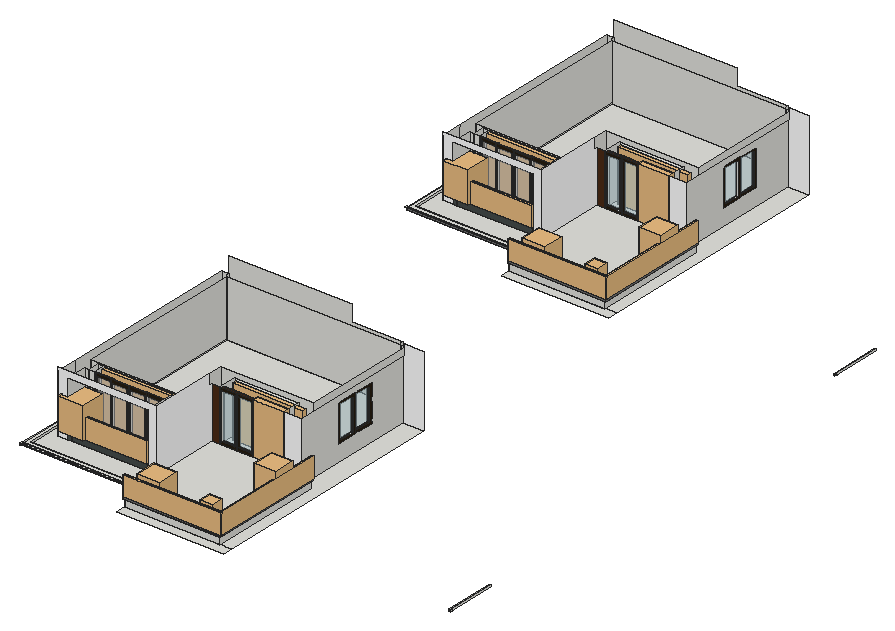
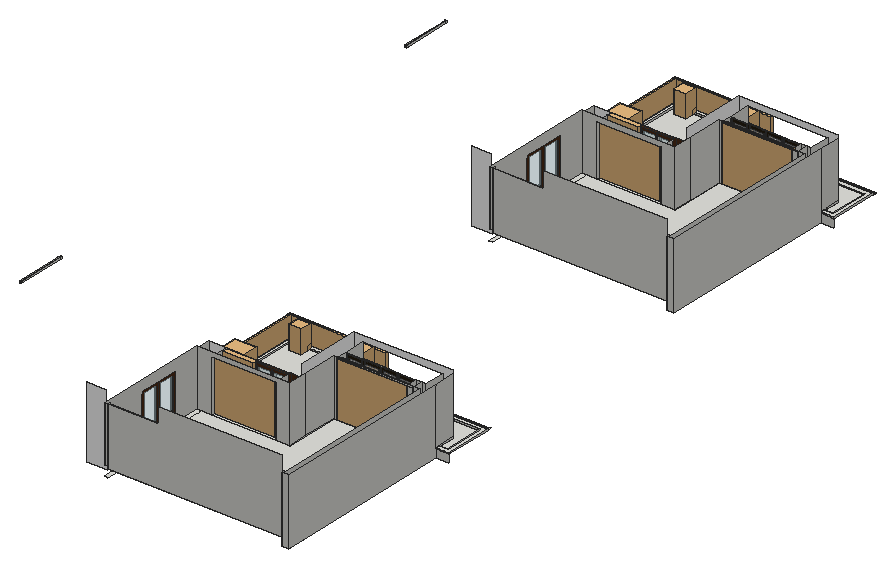
# SketchUp Ruby script. Lengths in inches.
U = 1.inch
M = Sketchup.active_model
def pt(a) = Geom::Point3d.new(a.map { |v| v * U })
def face(e, loops, mat)
  f = e.add_face(loops[0].map { |a| pt(a) })
  loops[1..].each { |l| e.add_face(l.map { |a| pt(a) }).erase! }
  f.material = f.back_material = mat if mat
  f
end
# faces: each face lists its corners as indices into pts; further lists are holes
def faces(e, pts, list, mat = nil) = list.each { |f| face(e, (f[0].is_a?(Array) ? f : [f]).map { |l| l.map { |i| pts[i] } }, mat) }
# xy, xz, yz: faces in a plane at the given z, y or x. An outline is a flat list of corners, or four numbers for a rectangle; further outlines are holes
def ring(l) = l.size == 4 ? [[l[0], l[1]], [l[2], l[1]], [l[2], l[3]], [l[0], l[3]]] : l.each_slice(2).to_a
def flat(e, list, mat, &to3) = list.each { |f| face(e, (f[0].is_a?(Array) ? f : [f]).map { |l| ring(l).map { |u, v| to3.(u, v) } }, mat) }
def xy(e, z, list, mat = nil) = flat(e, list, mat) { |x, y| [x, y, z] }
def xz(e, y, list, mat = nil) = flat(e, list, mat) { |x, z| [x, y, z] }
def yz(e, x, list, mat = nil) = flat(e, list, mat) { |y, z| [x, y, z] }
def lines(e, pts, list) = list.each { |a, b| e.add_line(pt(pts[a]), pt(pts[b])) }
# prism: a flat outline (further loops are holes) pulled along v
def prism(e, loops, v, mat = nil)
  f = face(e, loops, mat); d = Geom::Vector3d.new(v.map { |x| x * U })
  f.pushpull(f.normal.samedirection?(d) ? d.length : -d.length)
end
def box(e, o, s, mat = nil) = prism(e, [[o, [o[0] + s[0], o[1], o[2]], [o[0] + s[0], o[1] + s[1], o[2]], [o[0], o[1] + s[1], o[2]]]], [0, 0, s[2]], mat)
def at(x, y, z, deg = 0) = Geom::Transformation.translation(pt([x, y, z])) * Geom::Transformation.rotation(ORIGIN, Z_AXIS, deg.degrees)
def axes(o, x, y, z) = Geom::Transformation.new([*x, 0, *y, 0, *z, 0, *pt(o).to_a, 1])
def part(name) = M.definitions.add(name)
# library, detail: a bought-in or finely detailed component or shape, given as its bounding box
def library(name, o, s) = part(name).tap { |d| box(d.entities, o, s) }
def detail(e, o, s) = box(e.add_group.entities, o, s)
def put(e, d, t, mat = nil) = e.add_instance(d, t).tap { |i| i.material = mat if mat }
def group(e, t, mat = nil) = e.add_group.tap { |g| g.transformation = t; g.material = mat if mat }.entities
root = M.entities
M.materials.add("[Color M00]").color = [255, 255, 255]
M.materials.add("[Color M05]").color = [114, 114, 114]
M.materials.add("[Slate]").color = [70, 76, 75]
M.materials.add("[Translucent Glass Gray]2").color = [201, 201, 201]
M.materials["[Translucent Glass Gray]2"].alpha = 0.5
M.materials.add("[Translucent Glass Safety]").color = [204, 235, 244]
M.materials["[Translucent Glass Safety]"].alpha = 0.5
M.materials.add("[Wood Veneer 01]").color = [76, 44, 23]
M.materials.add("oak swatch").color = [40, 31, 19]
c1 = library("plant (1)",[-35.72,-28.42,0],[66.31,67.39,84.38])
c2 = library("Glass Railing",[0,0,0],[139.5,4.76,42])
c3 = part("Group\#6")
box(c3.entities,[0,0,0],[1.77,4.72,80.31],"oak swatch")
c4 = part("Exterior Sliding Doors")
xy(c4.entities,0,[[1.77,33.07,3.54,70.87],[1.77,70.87,3.54,108.66]])
xy(c4.entities,0,[[0,0,1.77,33.07],[0,108.66,1.77,141.73]],"oak swatch")
xy(c4.entities,4.72,[[0,4.72,1.77,33.07],[1.77,37.8,3.54,66.14],[1.77,75.88,3.54,103.9375],[0,108.66,1.77,137.01]],"oak swatch")
xy(c4.entities,75.59,[[1.77,37.8,3.54,66.14],[1.77,75.88,3.54,103.9375]])
xy(c4.entities,75.59,[[0,4.72,1.77,33.07],[0,108.66,1.77,137.01]],"oak swatch")
xy(c4.entities,80.31,[[0,0,1.77,33.07],[1.77,33.07,3.54,70.87],[1.77,70.87,3.54,108.66],[0,108.66,1.77,141.73]],"oak swatch")
xz(c4.entities,0,[[0,0,1.77,80.31]],"oak swatch")
xz(c4.entities,4.72,[[0,4.72,1.77,75.59]],"oak swatch")
xz(c4.entities,33.07,[[0,0,1.77,4.72],[1.77,0,3.54,80.31],[0,75.59,1.77,80.31]],"oak swatch")
xz(c4.entities,37.8,[[1.77,4.72,3.54,75.59]])
xz(c4.entities,66.14,[[1.77,4.72,3.54,75.59]],"oak swatch")
xz(c4.entities,70.87,[[1.77,0,3.54,80.31]])
xz(c4.entities,75.88,[[1.77,4.72,3.54,75.59]])
xz(c4.entities,103.9375,[[1.77,4.72,3.54,75.59]],"oak swatch")
xz(c4.entities,108.66,[[1.77,4.72,3.54,75.59]])
xz(c4.entities,108.66,[[0,0,3.54,4.72],[0,75.59,3.54,80.31]],"oak swatch")
xz(c4.entities,137.01,[[0,4.72,1.77,75.59]],"oak swatch")
xz(c4.entities,141.73,[[0,0,1.77,80.31]],"oak swatch")
yz(c4.entities,0,[[0,0,33.07,0,33.07,4.72,4.72,4.72,4.72,75.59,33.07,75.59,33.07,80.31,0,80.31],[108.66,0,141.73,0,141.73,80.31,108.66,80.31,108.66,75.59,137.01,75.59,137.01,4.72,108.66,4.72]],"oak swatch")
yz(c4.entities,1.77,[[4.72,4.72,33.07,75.59],[37.8,4.72,66.14,75.59],[75.88,4.72,103.9375,75.59],[108.66,4.72,137.01,75.59]],"[Translucent Glass Gray]2")
yz(c4.entities,1.77,[[0,0,33.07,0,33.07,4.72,4.72,4.72,4.72,75.59,33.07,75.59,33.07,80.31,0,80.31],[[33.07,0,70.87,80.31],[37.8,4.72,66.14,75.59]],[[70.87,0,141.73,80.31],[108.66,4.72,137.01,75.59],[75.88,4.72,103.9375,75.59]]],"oak swatch")
yz(c4.entities,3.54,[[[33.07,0,70.87,80.31],[37.8,4.72,66.14,75.59]],[[70.87,0,108.66,80.31],[75.88,4.72,103.9375,75.59]]],"oak swatch")
put(c4.entities,c3,at(0,33.07,0))
put(c4.entities,c3,at(0,103.9375,0))
c5 = library("Curtains",[0,0,0],[121.73,8.19,117.22])
c6 = library("Plant",[0,0,0],[12.59,12.59,14.16])
c7 = part("Group\#4")
g1 = group(c7.entities,at(0,0,0))
xy(g1,0,[[0,0,6,48]],"[Wood Veneer 01]")
xy(g1,4,[[0,4,1.8125,44],[1.8125,4,6,44]])
xy(g1,80,[[0,4,1.8125,44],[1.8125,4,6,44]])
xy(g1,84,[[0,0,6,48]],"[Wood Veneer 01]")
xz(g1,0,[[0,0,6,84]],"[Wood Veneer 01]")
xz(g1,4,[[0,4,1.8125,80],[1.8125,4,6,80]])
xz(g1,44,[[0,4,1.8125,80],[1.8125,4,6,80]])
xz(g1,48,[[0,0,6,84]],"[Wood Veneer 01]")
yz(g1,0,[[[0,0,48,84],[4,4,44,80]]],"[Wood Veneer 01]")
yz(g1,1.8125,[[4,4,44,80]],"[Translucent Glass Safety]")
yz(g1,6,[[[0,0,48,84],[4,4,44,80]]],"oak swatch")
g2 = group(c7.entities,at(0,48,0),"oak swatch")
xy(g2,0,[[0,0,6,48]],"[Wood Veneer 01]")
xy(g2,4,[[0,4,1.8125,44],[1.8125,4,6,44]])
xy(g2,80,[[0,4,1.8125,44],[1.8125,4,6,44]])
xy(g2,84,[[0,0,6,48]],"[Wood Veneer 01]")
xz(g2,0,[[0,0,6,84]],"[Wood Veneer 01]")
xz(g2,4,[[0,4,1.8125,80],[1.8125,4,6,80]])
xz(g2,44,[[0,4,1.8125,80],[1.8125,4,6,80]])
xz(g2,48,[[0,0,6,84]],"[Wood Veneer 01]")
yz(g2,0,[[[0,0,48,84],[4,4,44,80]]],"[Wood Veneer 01]")
yz(g2,1.8125,[[4,4,44,80]],"[Translucent Glass Safety]")
yz(g2,6,[[[0,0,48,84],[4,4,44,80]]],"oak swatch")
c8 = library("Flora+17",[-57.52,158.6,-38.64],[66.99,62.88,77.28])
c9 = library("modern+door",[0,0,0],[59.06,11.8125,86.61])
c10 = library("plant1",[-367.84,-375.82,-125.45],[750.59,696.16,1346.74])
c11 = part("skp4FF")
put(c11.entities,c10,at(0,0,0))
xy(root,121.3125,[[1384.3,481.81,1607.7,502.24],[1384.3,502.24,1583.39,538.49],[1583.39,502.24,1607.7,502.24,1607.7,1001.66,1563.95,1001.66,1563.95,738.06,1583.39,738.06],[1384.3,538.49,1583.39,638.99],[1172.33,638.99,1172.33,1021.31,1187.0625,1021.31,1187.0625,662.52,1204.64,662.52,1204.64,638.99],
  [1384.3,638.99,1583.39,738.06],[1204.64,648.22,1204.64,662.52,1364.27,662.52,1364.27,776.62,1373.95,776.62,1373.95,648.22],[1384.3,738.06,1563.95,749.87],[1548.25,813.85,1554.73,1021.31],[1384.3,1481.16,1607.7,1501.6],
  [1384.3,1501.6,1583.39,1537.85],[1583.39,1501.6,1607.7,1501.6,1607.7,2001.02,1563.95,2001.02,1563.95,1737.41,1583.39,1737.41],[1384.3,1537.85,1583.39,1638.35],[1172.33,1638.35,1172.33,2020.66,1187.0625,2020.66,1187.0625,1661.875,1204.64,1661.875,1204.64,1638.35],[1384.3,1638.35,1583.39,1737.41],
  [1204.64,1647.57,1204.64,1661.875,1364.27,1661.875,1364.27,1775.97,1373.95,1775.97,1373.95,1647.57],[1384.3,1737.41,1563.95,1749.22],[1548.25,1813.21,1554.73,2020.66]])
xy(root,138.1875,[[1384.3,497.56,1583.39,502.24],[1583.39,497.56,1588.08,502.24],[1384.3,502.24,1384.3,538.49,1145.33,538.49,1145.33,638.99,1172.33,638.99,1172.33,630.62,1153.58,630.62,1153.58,547.12,1390.64,547.12,1390.64,510.06,1577.08,510.06,1577.08,724.25,1563.95,724.25,1563.95,738.06,1583.39,738.06,1583.39,502.24],[1583.39,502.24,1588.08,738.06],[1390.64,510.06,1577.08,510.06,1577.08,724.25,1563.95,724.25,1563.95,738.06,1376.89,738.06,1376.89,595.06,1172.33,595.06,1172.33,630.62,1153.58,630.62,1153.58,547.12,1390.64,547.12],
  [1142.02,533.81,1145.33,538.49],[1145.33,533.81,1384.3,538.49],[1145.14,538.49,1145.33,638.99],[1172.33,595.06,1201.55,595.06,1201.55,606.41,1192.17,606.41,1192.17,638.99,1172.33,638.99],[1358.73,595.06,1376.89,638.99],
  [1192.17,606.41,1358.73,638.99],[1201.55,638.99,1213.92,662.52],[1213.92,638.99,1358.73,662.52],[1187.0625,662.52,1364.27,662.52,1364.27,776.62,1548.25,776.62,1548.25,1014.93,1187.0625,1014.93],[1394.93,738.06,1527.25,776.62],
  [1548.25,776.62,1558.25,1014.93],[1187.0625,1014.93,1548.25,1021.31],[1384.3,1496.91,1583.39,1501.6],[1583.39,1496.91,1588.08,1501.6],[1384.3,1501.6,1384.3,1537.85,1145.33,1537.85,1145.33,1638.35,1172.33,1638.35,1172.33,1629.97,1153.58,1629.97,1153.58,1546.47,1390.64,1546.47,1390.64,1509.41,1577.08,1509.41,1577.08,1723.61,1563.95,1723.61,1563.95,1737.41,1583.39,1737.41,1583.39,1501.6],
  [1583.39,1501.6,1588.08,1737.41],[1390.64,1509.41,1577.08,1509.41,1577.08,1723.61,1563.95,1723.61,1563.95,1737.41,1376.89,1737.41,1376.89,1594.41,1172.33,1594.41,1172.33,1629.97,1153.58,1629.97,1153.58,1546.47,1390.64,1546.47],[1145.33,1533.16,1384.3,1537.85],[1145.14,1537.85,1145.33,1638.35],[1172.33,1594.41,1201.55,1594.41,1201.55,1605.76,1192.17,1605.76,1192.17,1638.35,1172.33,1638.35],
  [1358.73,1594.41,1376.89,1638.35],[1192.17,1605.76,1358.73,1638.35],[1201.55,1638.35,1213.92,1661.875],[1213.92,1638.35,1358.73,1661.875],[1187.0625,1661.875,1364.27,1661.875,1364.27,1775.97,1548.25,1775.97,1548.25,2014.29,1187.0625,2014.29],
  [1394.93,1737.41,1527.25,1775.97],[1548.25,1775.97,1558.25,2014.29],[1187.0625,2014.29,1548.25,2020.66]])
xy(root,141.4375,[[1384.3,497.56,1588.08,497.56,1588.08,738.06,1583.39,738.06,1583.39,502.24,1384.3,502.24],[1384.3,502.24,1583.39,502.24,1583.39,738.06,1563.95,738.06,1563.95,724.25,1577.08,724.25,1577.08,510.06,1390.64,510.06,1390.64,547.12,1153.58,547.12,1153.58,630.62,1172.33,630.62,1172.33,638.99,1145.33,638.99,1145.33,538.49,1384.3,538.49],[1142.02,533.81,1145.33,538.49],[1145.33,533.81,1384.3,538.49],[1145.14,538.49,1145.33,638.99],
  [1384.3,1496.91,1588.08,1496.91,1588.08,1737.41,1583.39,1737.41,1583.39,1501.6,1384.3,1501.6],[1384.3,1501.6,1583.39,1501.6,1583.39,1737.41,1563.95,1737.41,1563.95,1723.61,1577.08,1723.61,1577.08,1509.41,1390.64,1509.41,1390.64,1546.47,1153.58,1546.47,1153.58,1629.97,1172.33,1629.97,1172.33,1638.35,1145.33,1638.35,1145.33,1537.85,1384.3,1537.85],[1142.02,1533.16,1145.33,1537.85],[1145.33,1533.16,1384.3,1537.85],[1145.14,1537.85,1145.33,1638.35]])
xy(root,142.875,[[2034.61,531.5,2037.92,536.1875],[2034.61,536.1875,2037.73,636.6875],[2037.73,536.1875,2037.92,636.6875],[2034.61,1530.85,2037.92,1535.54],[2034.61,1535.54,2037.73,1636.04],
  [2037.73,1535.54,2037.92,1636.04]])
xy(root,146.125,[[2034.61,531.5,2037.92,536.1875],[2034.61,536.1875,2037.73,636.6875],[2037.73,536.1875,2037.92,636.6875],[2034.61,1530.85,2037.92,1535.54],[2034.61,1535.54,2037.73,1636.04],
  [2037.73,1535.54,2037.92,1636.04]])
xy(root,152,[[1192.17,595.06,1201.55,606.41],[1201.55,595.06,1358.73,606.41],[1192.17,1594.41,1201.55,1605.76],[1201.55,1594.41,1358.73,1605.76]],"[Slate]")
xy(root,155.89,[[1558.25,833.57,1563.95,919.13],[1558.25,1832.92,1563.95,1918.48]])
xz(root,497.56,[[1384.3,138.1875,1588.08,141.4375]],"[Color M05]")
xz(root,502.24,[[1384.3,121.3125,1583.39,138.1875],[1384.3,138.1875,1583.39,141.4375]])
xz(root,510.06,[[1390.64,138.1875,1577.08,141.4375]])
xz(root,531.5,[[2034.61,142.875,2037.92,146.125]])
xz(root,533.81,[[1145.33,138.1875,1384.3,141.4375]],"[Color M05]")
xz(root,536.1875,[[2034.61,142.875,2037.73,146.125],[2037.73,142.875,2037.92,146.125]])
xz(root,538.49,[[1145.14,138.1875,1145.33,141.4375],[1145.33,138.1875,1384.3,141.4375]])
xz(root,547.12,[[1153.58,138.1875,1390.64,141.4375]])
xz(root,595.06,[[1172.33,138.1875,1192.17,138.1875,1192.17,252.5,1358.73,252.5,1358.73,138.1875,1376.89,138.1875,1376.89,265.6875,1172.33,265.6875]],"[Color M00]")
xz(root,595.06,[[1192.17,138.1875,1201.55,152],[1201.55,138.1875,1358.73,152]],"[Slate]")
xz(root,606.41,[[1192.17,138.1875,1201.55,152],[1201.55,138.1875,1358.73,152]])
xz(root,630.62,[[1153.58,138.1875,1172.33,141.4375]])
xz(root,636.6875,[[2034.61,142.875,2037.73,146.125],[2037.73,142.875,2037.92,146.125]])
xz(root,638.99,[[1145.33,121.3125,1172.33,138.1875],[1145.14,138.1875,1145.33,141.4375],[1145.33,138.1875,1172.33,141.4375],[1192.17,138.1875,1201.55,252.5],[1201.55,138.1875,1213.92,252.5]])
xz(root,662.52,[[1187.0625,121.3125,1364.27,138.1875],[1187.0625,138.1875,1187.0625,254.625,1364.27,254.625,1364.27,138.1875,1358.73,138.1875,1358.73,252.5,1201.55,252.5,1201.55,138.1875],[1201.55,138.1875,1213.92,252.5]])
xz(root,724.25,[[1563.95,138.1875,1577.08,141.4375]])
xz(root,738.06,[[1563.95,121.3125,1583.39,138.1875],[1563.95,138.1875,1583.39,141.4375],[1583.39,138.1875,1588.08,141.4375]])
xz(root,738.06,[[1527.25,138.1875,1563.95,244.75]],"[Color M00]")
xz(root,738.06,[[1376.89,138.1875,1394.93,244.75]],"[Wood Veneer 01]")
xz(root,776.62,[[1364.27,138.1875,1364.27,254.625,1558.25,254.625,1558.25,138.1875,1527.25,138.1875,1527.25,244.75,1394.93,244.75,1394.93,138.1875]])
xz(root,833.57,[[1558.25,155.89,1563.95,232.14]])
xz(root,919.13,[[1558.25,155.89,1563.95,232.14]])
xz(root,1001.66,[[1563.95,121.3125,1607.7,121.3125,1607.7,269.375,1567.08,269.375,1567.08,244.75,1563.95,244.75]],"[Color M00]")
xz(root,1014.93,[[1187.0625,138.1875,1548.25,254.625],[1548.25,138.1875,1558.25,254.625]])
xz(root,1021.31,[[1172.33,121.3125,1187.0625,258.1875],[1187.0625,138.1875,1187.0625,291.125,1440.7,291.125,1440.7,258.1875,1548.25,258.1875,1548.25,138.1875]])
xz(root,1496.91,[[1384.3,138.1875,1588.08,141.4375]],"[Color M05]")
xz(root,1501.6,[[1384.3,121.3125,1583.39,138.1875],[1384.3,138.1875,1583.39,141.4375]])
xz(root,1509.41,[[1390.64,138.1875,1577.08,141.4375]])
xz(root,1530.85,[[2034.61,142.875,2037.92,146.125]])
xz(root,1533.16,[[1145.33,138.1875,1384.3,141.4375]],"[Color M05]")
xz(root,1535.54,[[2034.61,142.875,2037.73,146.125],[2037.73,142.875,2037.92,146.125]])
xz(root,1537.85,[[1145.14,138.1875,1145.33,141.4375],[1145.33,138.1875,1384.3,141.4375]])
xz(root,1546.47,[[1153.58,138.1875,1390.64,141.4375]])
xz(root,1594.41,[[1172.33,138.1875,1192.17,138.1875,1192.17,252.5,1358.73,252.5,1358.73,138.1875,1376.89,138.1875,1376.89,265.6875,1172.33,265.6875]],"[Color M00]")
xz(root,1594.41,[[1192.17,138.1875,1201.55,152],[1201.55,138.1875,1358.73,152]],"[Slate]")
xz(root,1605.76,[[1192.17,138.1875,1201.55,152],[1201.55,138.1875,1358.73,152]])
xz(root,1629.97,[[1153.58,138.1875,1172.33,141.4375]])
xz(root,1636.04,[[2034.61,142.875,2037.73,146.125],[2037.73,142.875,2037.92,146.125]])
xz(root,1638.35,[[1145.33,121.3125,1172.33,138.1875],[1145.14,138.1875,1145.33,141.4375],[1145.33,138.1875,1172.33,141.4375],[1192.17,138.1875,1201.55,252.5],[1201.55,138.1875,1213.92,252.5]])
xz(root,1661.875,[[1187.0625,121.3125,1364.27,138.1875],[1187.0625,138.1875,1187.0625,254.625,1364.27,254.625,1364.27,138.1875,1358.73,138.1875,1358.73,252.5,1201.55,252.5,1201.55,138.1875],[1201.55,138.1875,1213.92,252.5]])
xz(root,1723.61,[[1563.95,138.1875,1577.08,141.4375]])
xz(root,1737.41,[[1563.95,121.3125,1583.39,138.1875],[1563.95,138.1875,1583.39,141.4375],[1583.39,138.1875,1588.08,141.4375]])
xz(root,1737.41,[[1527.25,138.1875,1563.95,244.75]],"[Color M00]")
xz(root,1737.41,[[1376.89,138.1875,1394.93,244.75]],"[Wood Veneer 01]")
xz(root,1775.97,[[1364.27,138.1875,1364.27,254.625,1558.25,254.625,1558.25,138.1875,1527.25,138.1875,1527.25,244.75,1394.93,244.75,1394.93,138.1875]])
xz(root,1832.92,[[1558.25,155.89,1563.95,232.14]])
xz(root,1918.48,[[1558.25,155.89,1563.95,232.14]])
xz(root,2001.02,[[1563.95,121.3125,1607.7,121.3125,1607.7,269.375,1567.08,269.375,1567.08,244.75,1563.95,244.75]],"[Color M00]")
xz(root,2014.29,[[1187.0625,138.1875,1548.25,254.625],[1548.25,138.1875,1558.25,254.625]])
xz(root,2020.66,[[1172.33,121.3125,1187.0625,258.1875],[1187.0625,138.1875,1187.0625,291.125,1440.7,291.125,1440.7,258.1875,1548.25,258.1875,1548.25,138.1875]])
yz(root,1145.14,[[538.49,138.1875,638.99,141.4375],[1537.85,138.1875,1638.35,141.4375]])
yz(root,1145.33,[[533.81,138.1875,538.49,141.4375],[538.49,138.1875,638.99,141.4375],[1533.16,138.1875,1537.85,141.4375],[1537.85,138.1875,1638.35,141.4375]])
yz(root,1153.58,[[547.12,138.1875,630.62,141.4375],[1546.47,138.1875,1629.97,141.4375]])
yz(root,1172.33,[[638.99,121.3125,1021.31,258.1875],[1638.35,121.3125,2020.66,258.1875],[595.06,138.1875,630.62,141.4375],[630.62,138.1875,638.99,141.4375],[1594.41,138.1875,1629.97,141.4375],
  [1629.97,138.1875,1638.35,141.4375],[595.06,141.4375,638.99,258.1875],[1594.41,141.4375,1638.35,258.1875]])
yz(root,1187.0625,[[662.52,121.3125,1021.31,138.1875],[1661.875,121.3125,2020.66,138.1875],[662.52,138.1875,1014.93,254.625],[1014.93,138.1875,1021.31,258.1875],[1661.875,138.1875,2014.29,254.625],
  [2014.29,138.1875,2020.66,258.1875]])
yz(root,1192.17,[[606.41,138.1875,638.99,138.1875,638.99,252.5,595.06,252.5,595.06,152,606.41,152],[1605.76,138.1875,1638.35,138.1875,1638.35,252.5,1594.41,252.5,1594.41,152,1605.76,152]])
yz(root,1201.55,[[595.06,138.1875,606.41,152],[638.99,138.1875,662.52,252.5],[1594.41,138.1875,1605.76,152],[1638.35,138.1875,1661.875,252.5]])
yz(root,1213.92,[[638.99,138.1875,662.52,252.5],[1638.35,138.1875,1661.875,252.5]])
yz(root,1358.73,[[595.06,138.1875,606.41,152],[606.41,138.1875,606.41,152,595.06,152,595.06,252.5,638.99,252.5,638.99,138.1875],[638.99,138.1875,662.52,252.5],[1594.41,138.1875,1605.76,152],[1605.76,138.1875,1605.76,152,1594.41,152,1594.41,252.5,1638.35,252.5,1638.35,138.1875],
  [1638.35,138.1875,1661.875,252.5]])
yz(root,1364.27,[[662.52,121.3125,738.06,138.1875],[738.06,121.3125,776.62,138.1875],[1661.875,121.3125,1737.41,138.1875],[1737.41,121.3125,1775.97,138.1875],[662.52,138.1875,738.06,254.625],
  [738.06,138.1875,776.62,254.625],[1661.875,138.1875,1737.41,254.625],[1737.41,138.1875,1775.97,254.625]])
yz(root,1376.89,[[595.06,138.1875,738.06,138.1875,738.06,244.75,731.24,244.75,731.24,265.6875,595.06,265.6875],[1594.41,138.1875,1737.41,138.1875,1737.41,244.75,1730.6,244.75,1730.6,265.6875,1594.41,265.6875]],"[Color M00]")
yz(root,1384.3,[[502.24,121.3125,538.49,138.1875],[1501.6,121.3125,1537.85,138.1875],[497.56,138.1875,502.24,141.4375],[502.24,138.1875,533.81,141.4375],[533.81,138.1875,538.49,141.4375],
  [1496.91,138.1875,1501.6,141.4375],[1501.6,138.1875,1533.16,141.4375],[1533.16,138.1875,1537.85,141.4375]])
yz(root,1390.64,[[510.06,138.1875,547.12,141.4375],[1509.41,138.1875,1546.47,141.4375]])
yz(root,1394.93,[[738.06,138.1875,776.62,244.75],[1737.41,138.1875,1775.97,244.75]])
yz(root,1527.25,[[738.06,138.1875,776.62,244.75],[1737.41,138.1875,1775.97,244.75]])
yz(root,1548.25,[[1014.93,138.1875,1021.31,258.1875],[2014.29,138.1875,2020.66,258.1875]])
yz(root,1558.25,[[[776.62,138.1875,1014.93,254.625],[833.57,155.89,919.13,232.14]],[[1775.97,138.1875,2014.29,254.625],[1832.92,155.89,1918.48,232.14]]])
yz(root,1563.95,[[[738.06,121.3125,1001.66,244.75],[833.57,155.89,919.13,232.14]],[[1737.41,121.3125,2001.02,244.75],[1832.92,155.89,1918.48,232.14]],[724.25,138.1875,738.06,141.4375],[1723.61,138.1875,1737.41,141.4375]])
yz(root,1577.08,[[510.06,138.1875,724.25,141.4375],[1509.41,138.1875,1723.61,141.4375]])
yz(root,1583.39,[[502.24,121.3125,738.06,138.1875],[1501.6,121.3125,1737.41,138.1875],[502.24,138.1875,738.06,141.4375],[1501.6,138.1875,1737.41,141.4375]])
yz(root,1588.08,[[497.56,138.1875,738.06,141.4375],[1496.91,138.1875,1737.41,141.4375]],"[Color M05]")
yz(root,2034.61,[[531.5,142.875,536.1875,146.125],[536.1875,142.875,636.6875,146.125],[1530.85,142.875,1535.54,146.125],[1535.54,142.875,1636.04,146.125]])
yz(root,2037.73,[[536.1875,142.875,636.6875,146.125],[1535.54,142.875,1636.04,146.125]])
yz(root,2037.92,[[531.5,142.875,536.1875,146.125],[536.1875,142.875,636.6875,146.125]])
put(root,c1,axes([1207.46,1607.49,153.49],[0.77,0,0],[0,0.77,0],[0,0,0.77]))
put(root,c1,axes([1207.46,608.13,153.49],[0.77,0,0],[0,0.77,0],[0,0,0.77]))
put(root,c2,axes([1192.17,1591.4375,152.79],[1.194,0,0],[0,1,0],[0,0,1]))
put(root,c2,axes([1192.17,592.08,152.79],[1.194,0,0],[0,1,0],[0,0,1]))
put(root,c4,axes([1214.9,1640.12,138.1875],[0,-1,0],[0.99858,0,0],[0,0,1.4151]))
put(root,c4,axes([1214.9,640.77,138.1875],[0,-1,0],[0.99858,0,0],[0,0,1.4151]))
put(root,c5,axes([1213.38,1653.68,138.1875],[1.19408,0,0],[0,1,0],[0,0,0.96546]))
put(root,c5,axes([1213.38,654.32,138.1875],[1.19408,0,0],[0,1,0],[0,0,0.96546]))
put(root,c6,axes([1400.98,1517.43,138.1875],[0.7,0,0],[0,0.7,0],[0,0,0.7]))
put(root,c6,axes([1400.98,518.07,138.1875],[0.7,0,0],[0,0.7,0],[0,0,0.7]))
put(root,c7,axes([1394.41,1743.41,138.1875],[0,-1,0],[0.71,0,0],[0,0,1.26]))
put(root,c7,axes([1394.41,744.06,138.1875],[0,-1,0],[0.71,0,0],[0,0,1.26]))
put(root,c8,axes([1447.17,1393.6875,160.89],[0.71,0,0],[0,0.71,0],[0,0,0.71]))
put(root,c8,axes([1447.17,394.33,160.89],[0.71,0,0],[0,0.71,0],[0,0,0.71]))
put(root,c5,axes([1401.98,1761.9,130.52],[1.19408,0,0],[0,1,0],[0,0,0.96546]))
put(root,c5,axes([1401.98,762.55,130.52],[1.19408,0,0],[0,1,0],[0,0,0.96546]))
put(root,c2,axes([1384.41,1496.91,141.4375],[1.46,0,0],[0,1,0],[0,0,1]))
put(root,c2,axes([1384.41,497.56,141.4375],[1.46,0,0],[0,1,0],[0,0,1]))
put(root,c9,axes([1462.875,1737.41,138.1875],[1.09,0,0],[0,1,0],[0,0,1.23031]))
put(root,c9,axes([1462.875,738.06,138.1875],[1.09,0,0],[0,1,0],[0,0,1.23031]))
put(root,c6,axes([1536.9375,1505.95,138.1875],[0.7,0,0],[0,0.7,0],[0,0,0.7]))
put(root,c6,axes([1536.9375,506.59,138.1875],[0.7,0,0],[0,0.7,0],[0,0,0.7]))
put(root,c11,axes([1550.42,1519.74,142.62],[0.03534,0,0],[0,0.03534,0],[0,0,0.03534]))
put(root,c11,axes([1550.42,520.38,142.62],[0.03534,0,0],[0,0.03534,0],[0,0,0.03534]))
put(root,c7,axes([1557.95,1832.92,155.89],[1,0,0],[0,0.88868,0],[0,0,0.90774]))
put(root,c7,axes([1557.95,833.57,155.89],[1,0,0],[0,0.88868,0],[0,0,0.90774]))
put(root,c1,axes([1567.59,1658.45,141.4375],[0.67,0,0],[0,0.67,0],[0,0,0.67]))
put(root,c1,axes([1567.59,659.09,141.4375],[0.67,0,0],[0,0.67,0],[0,0,0.67]))
put(root,c2,axes([1588.15,1499.92,141.41],[0,1.70244,0],[-1,0,0],[0,0,1]))
put(root,c2,axes([1588.15,500.57,141.41],[0,1.70244,0],[-1,0,0],[0,0,1]))
